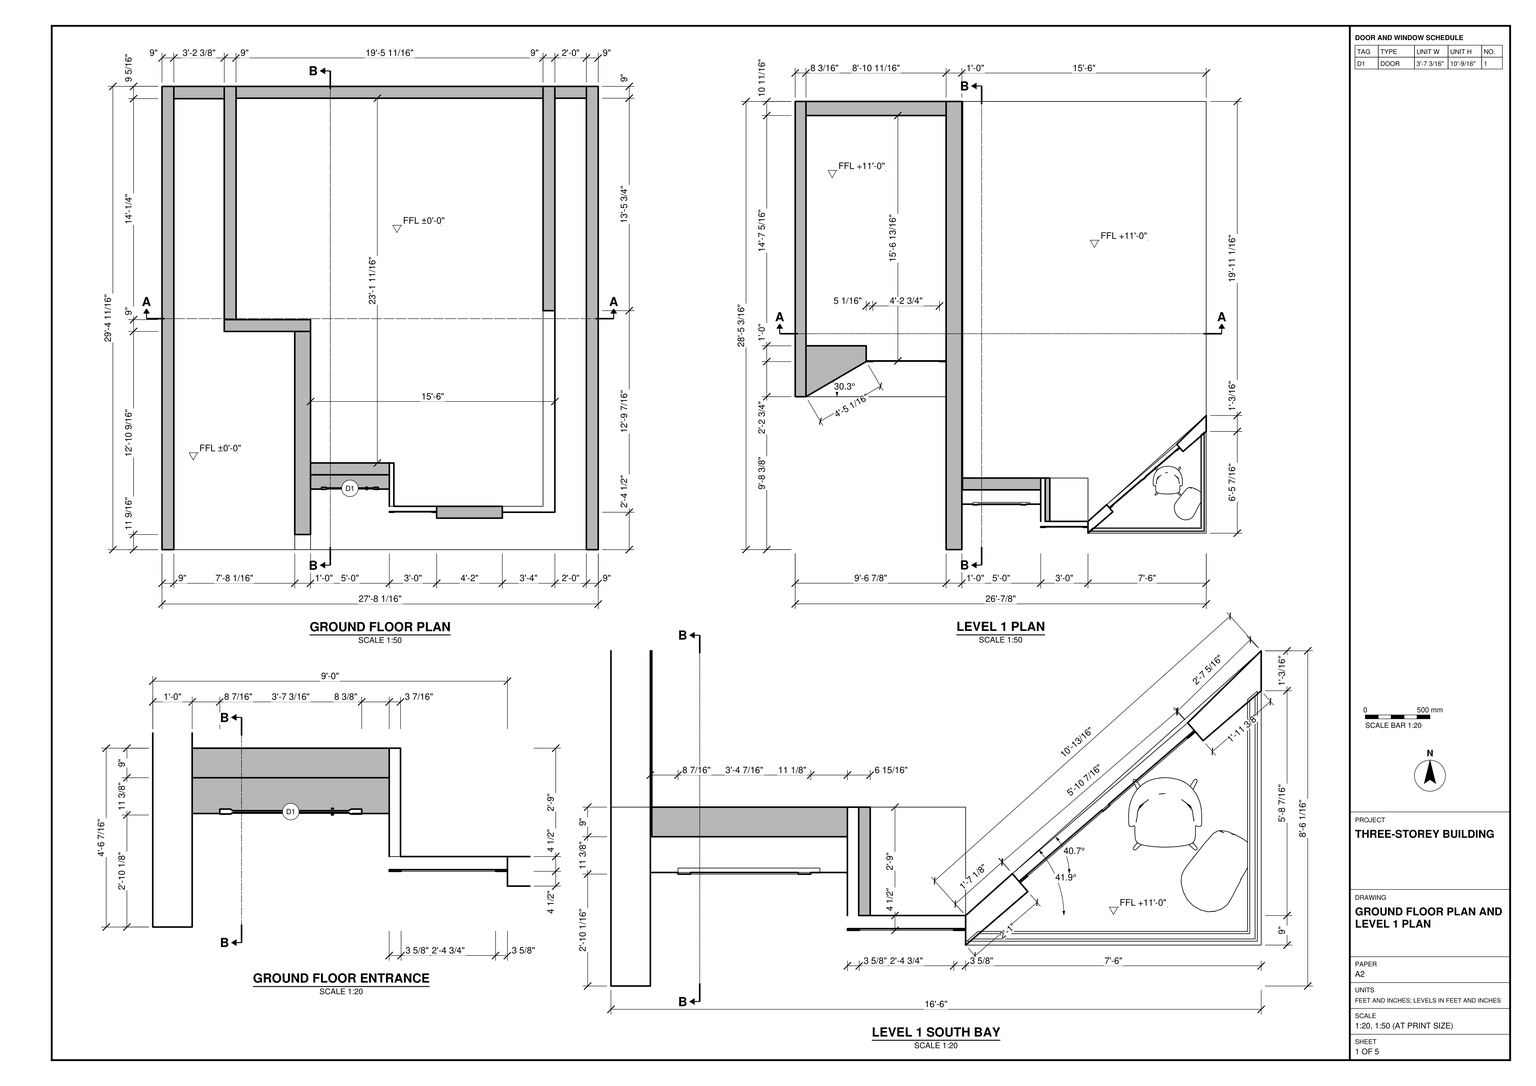
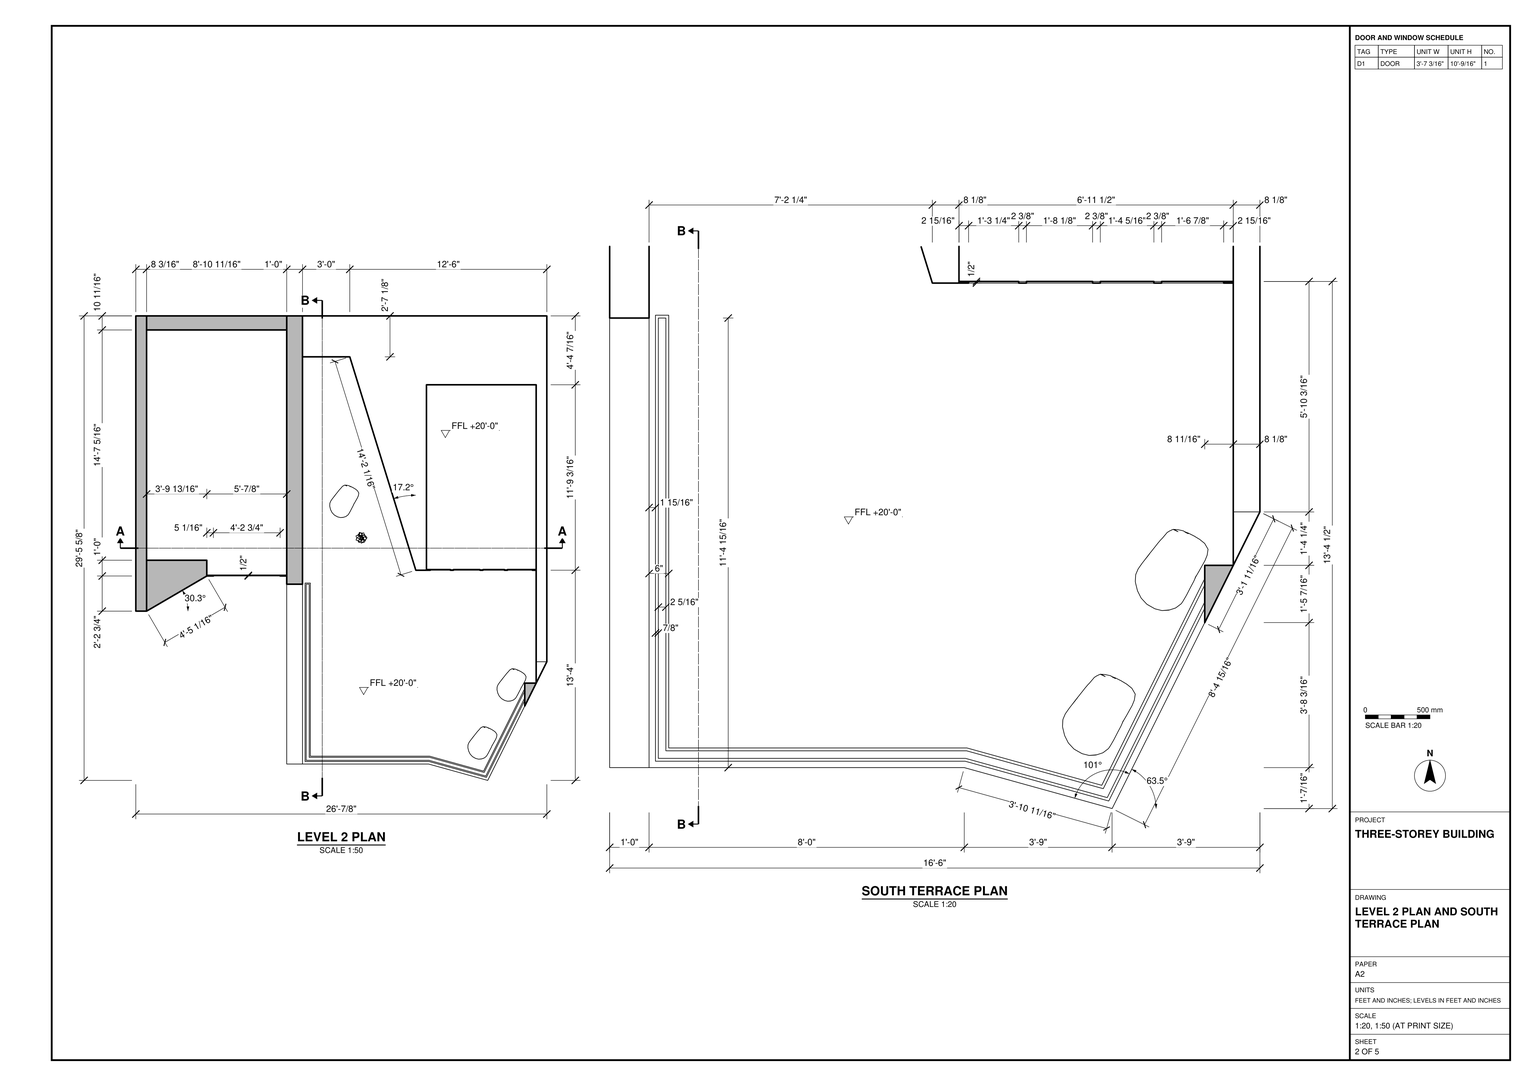
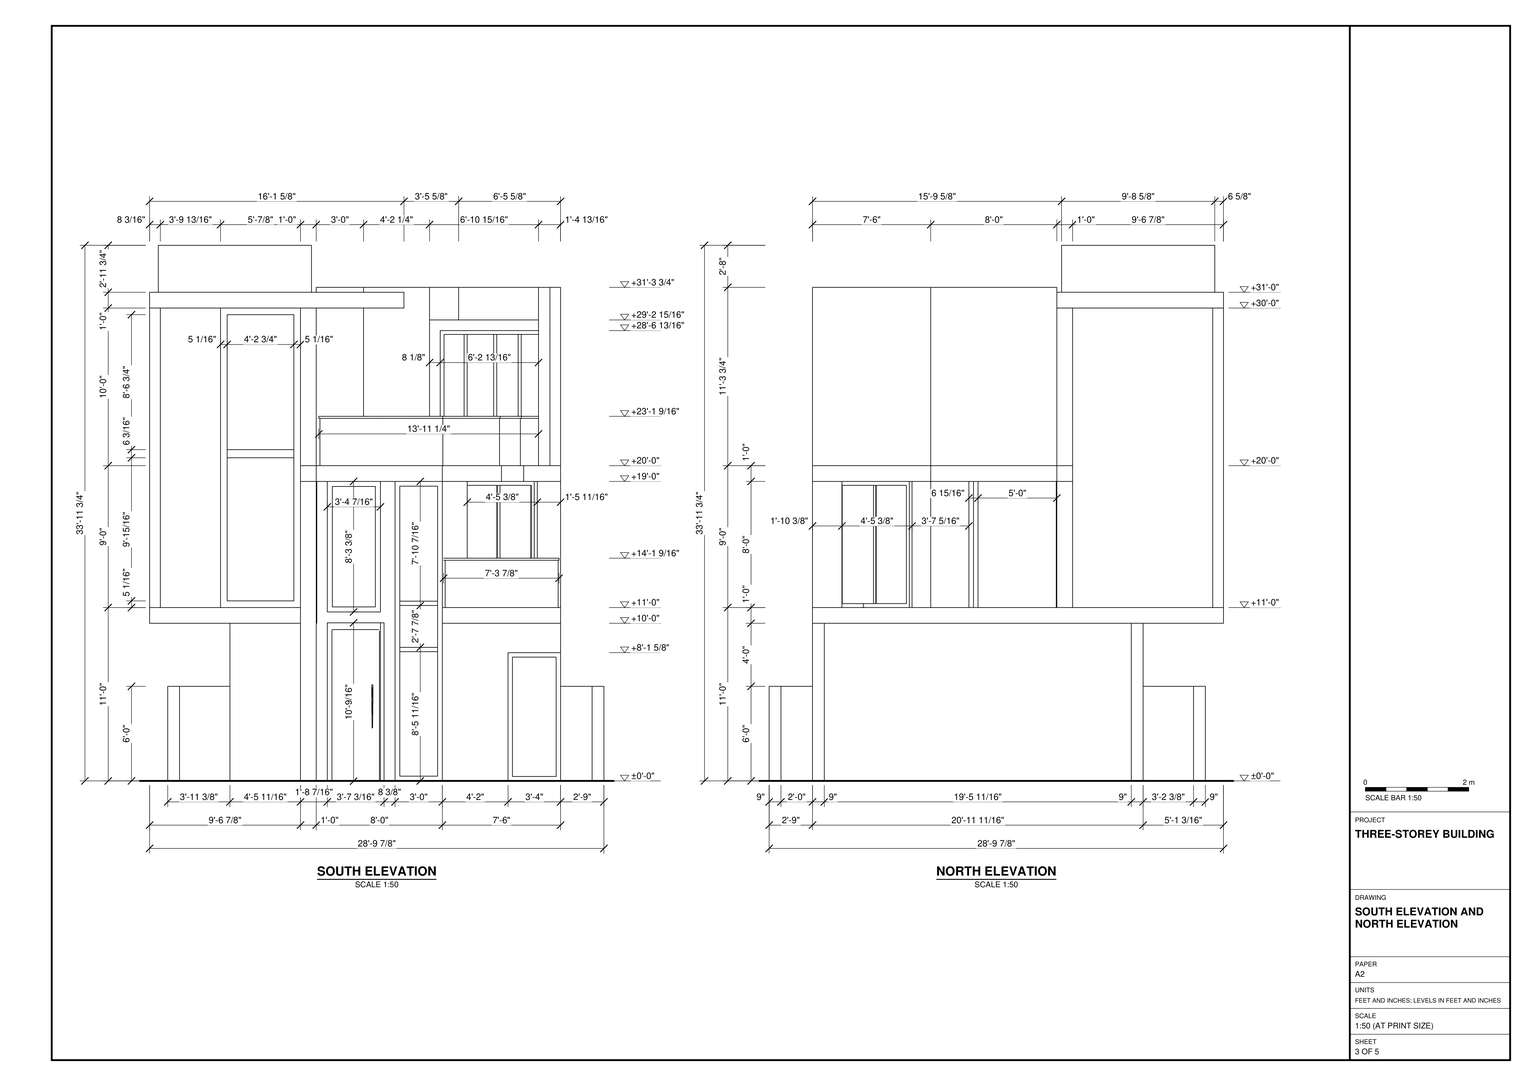
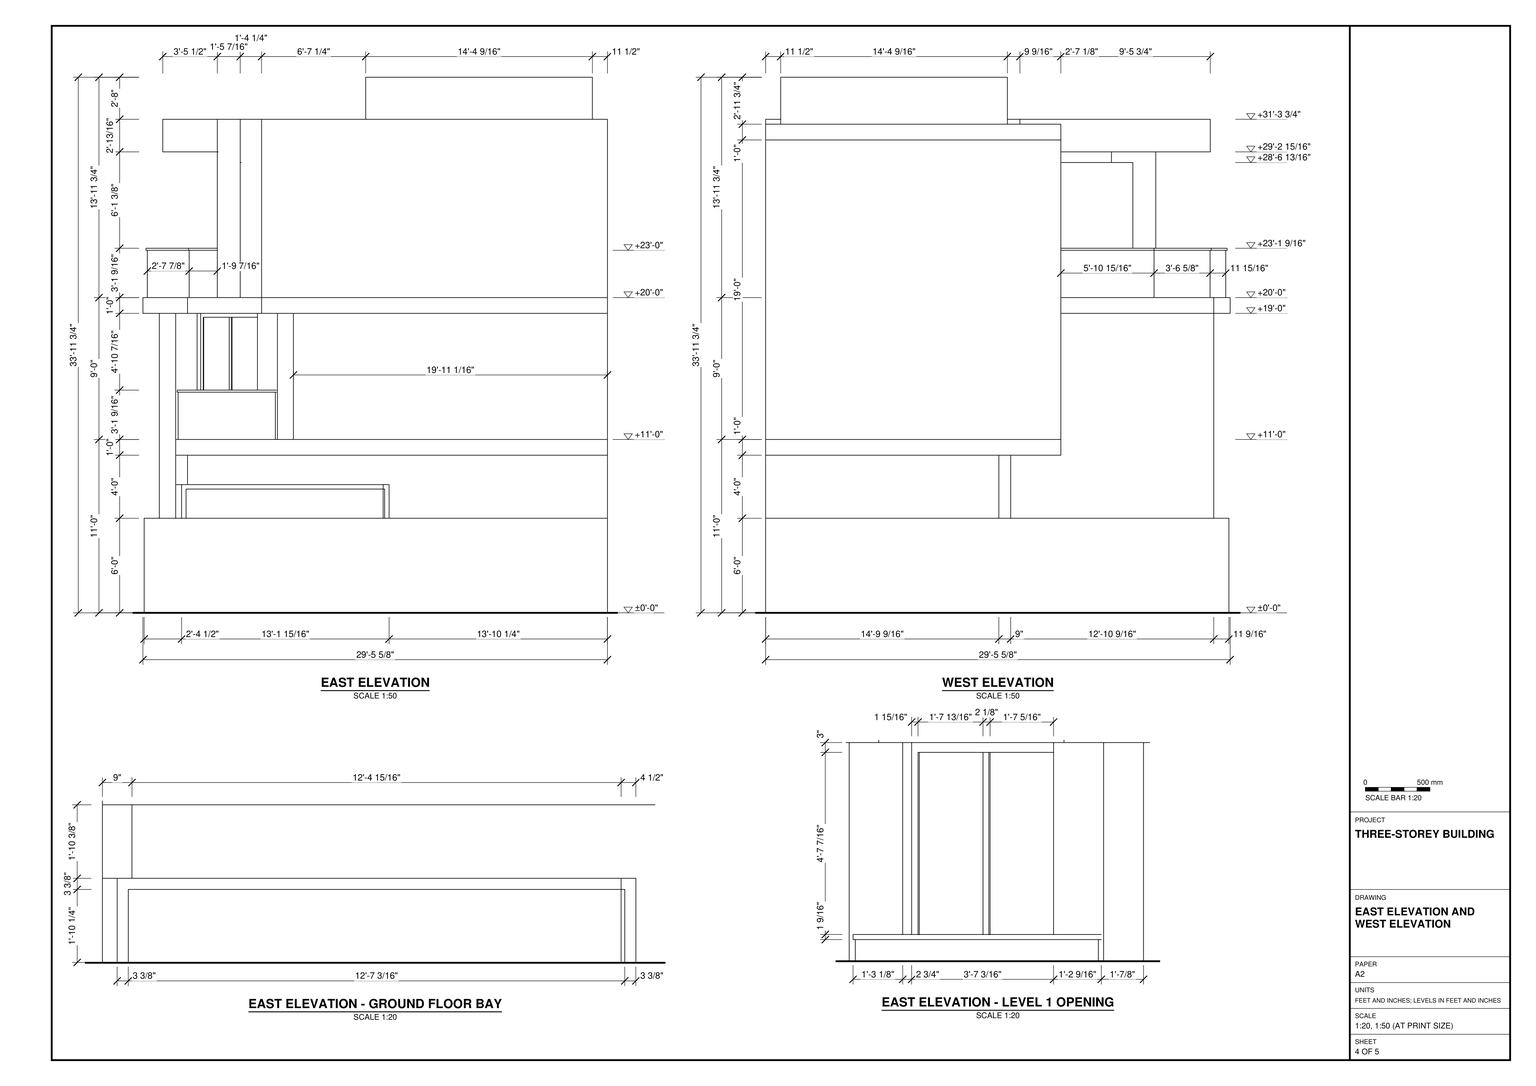
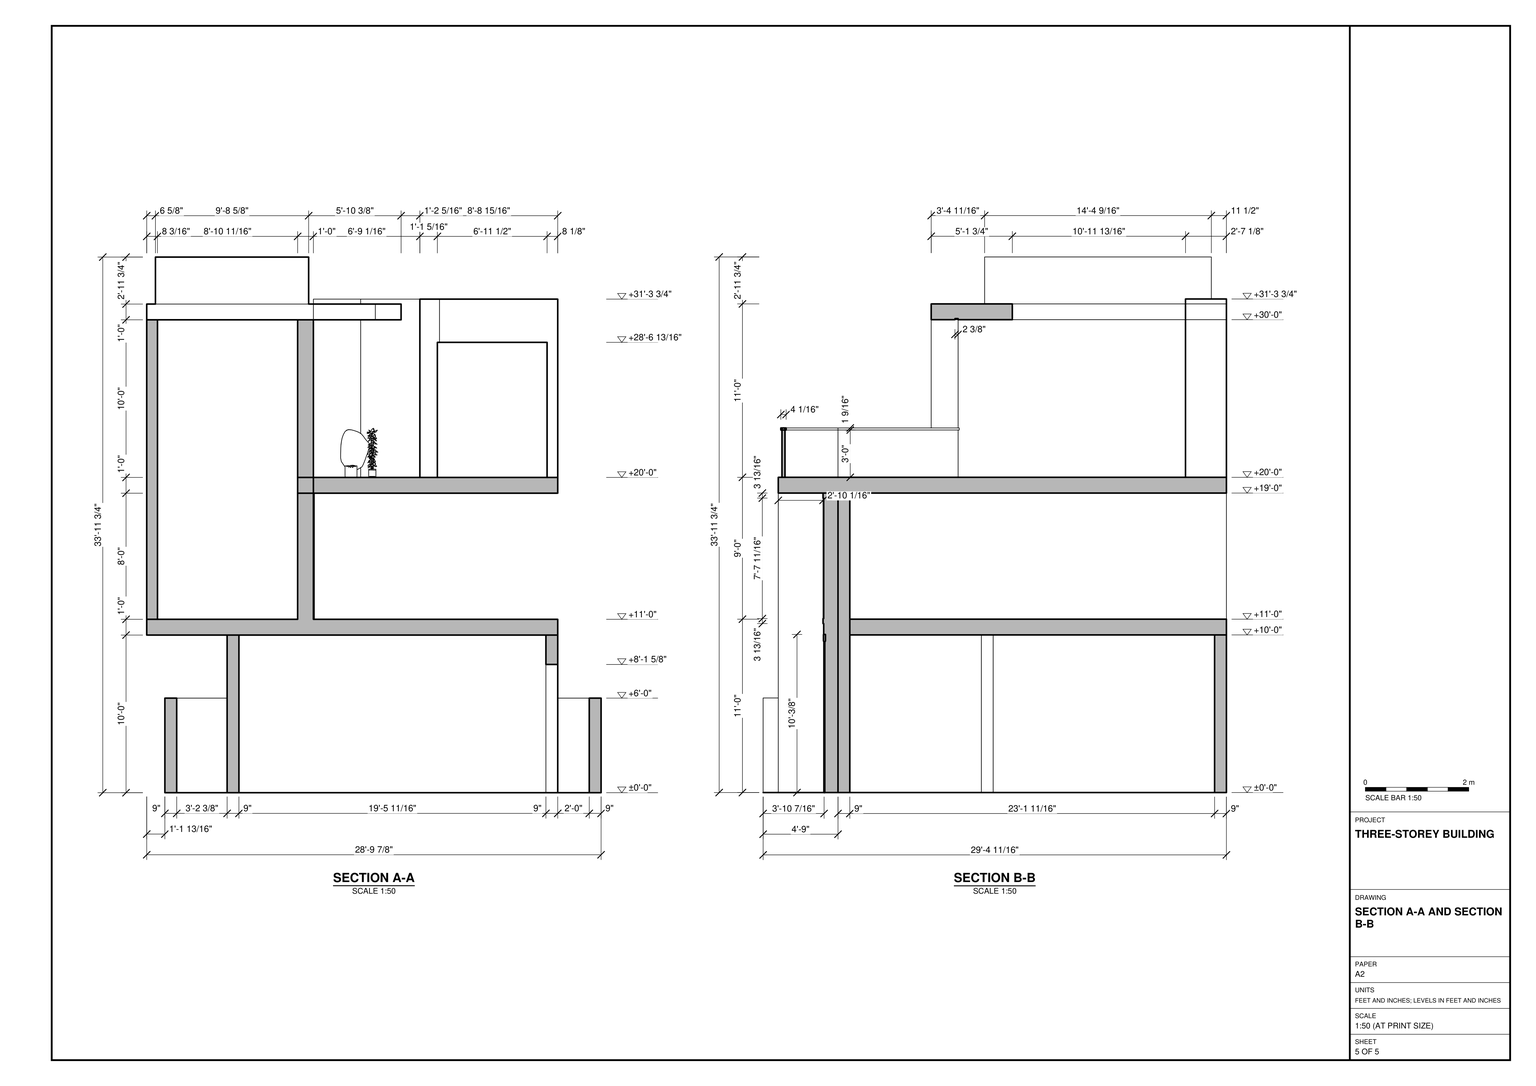
Build the three-storey building in SketchUp using task_files/diagram_01.pdf. Work in feet and inches. Set out the model with an overall width of 28'-9 7/8" along X, a depth of 29'-5 5/8" along Y and a height of 33'-11 15/16" along Z. Use finished floor levels of ±0'-0" for the ground floor, +11'-0" for Level 1 and +20'-0" for Level 2.

Follow the ground-floor plan for the long outer walls, the offset in the interior wall and the stepped south entrance. Use the wall thicknesses shown, including the 9" outer side walls at ground level. Fit the entrance door into its recess and use the elevations to align the framed openings with the slab edges. On Level 1, form the triangular south bay with its diagonal edge and seating. Above it, follow the Level 2 plan for the larger south terrace: its front edge changes direction before meeting the long angled side. Carry the terrace guard around those changes in direction. Model the flat roof sections at their different heights so the narrow western volume rises above the adjoining roof.

Keep walls, slabs, roof sections and each furniture or joinery piece in separate groups or components, and use components for repeated parts. Decor and loose items, including plants, may be any suitable library components. Save one SketchUp model as output_files/three_storey_building_with_a_faceted_south_terrace.skp.

# SketchUp Ruby script. Lengths in inches.
U = 1.inch
M = Sketchup.active_model
def pt(a) = Geom::Point3d.new(a.map { |v| v * U })
def face(e, loops, mat)
  f = e.add_face(loops[0].map { |a| pt(a) })
  loops[1..].each { |l| e.add_face(l.map { |a| pt(a) }).erase! }
  f.material = f.back_material = mat if mat
  f
end
# faces: each face lists its corners as indices into pts; further lists are holes
def faces(e, pts, list, mat = nil) = list.each { |f| face(e, (f[0].is_a?(Array) ? f : [f]).map { |l| l.map { |i| pts[i] } }, mat) }
# xy, xz, yz: faces in a plane at the given z, y or x. An outline is a flat list of corners, or four numbers for a rectangle; further outlines are holes
def ring(l) = l.size == 4 ? [[l[0], l[1]], [l[2], l[1]], [l[2], l[3]], [l[0], l[3]]] : l.each_slice(2).to_a
def flat(e, list, mat, &to3) = list.each { |f| face(e, (f[0].is_a?(Array) ? f : [f]).map { |l| ring(l).map { |u, v| to3.(u, v) } }, mat) }
def xy(e, z, list, mat = nil) = flat(e, list, mat) { |x, y| [x, y, z] }
def xz(e, y, list, mat = nil) = flat(e, list, mat) { |x, z| [x, y, z] }
def yz(e, x, list, mat = nil) = flat(e, list, mat) { |y, z| [x, y, z] }
def lines(e, pts, list) = list.each { |a, b| e.add_line(pt(pts[a]), pt(pts[b])) }
# prism: a flat outline (further loops are holes) pulled along v
def prism(e, loops, v, mat = nil)
  f = face(e, loops, mat); d = Geom::Vector3d.new(v.map { |x| x * U })
  f.pushpull(f.normal.samedirection?(d) ? d.length : -d.length)
end
def box(e, o, s, mat = nil) = prism(e, [[o, [o[0] + s[0], o[1], o[2]], [o[0] + s[0], o[1] + s[1], o[2]], [o[0], o[1] + s[1], o[2]]]], [0, 0, s[2]], mat)
def at(x, y, z, deg = 0) = Geom::Transformation.translation(pt([x, y, z])) * Geom::Transformation.rotation(ORIGIN, Z_AXIS, deg.degrees)
def axes(o, x, y, z) = Geom::Transformation.new([*x, 0, *y, 0, *z, 0, *pt(o).to_a, 1])
def part(name) = M.definitions.add(name)
# library, detail: a bought-in or finely detailed component or shape, given as its bounding box
def library(name, o, s) = part(name).tap { |d| box(d.entities, o, s) }
def detail(e, o, s) = box(e.add_group.entities, o, s)
def put(e, d, t, mat = nil) = e.add_instance(d, t).tap { |i| i.material = mat if mat }
def group(e, t, mat = nil) = e.add_group.tap { |g| g.transformation = t; g.material = mat if mat }.entities
root = M.entities
M.materials.add("[Color M06]").color = [86, 86, 86]
M.materials.add("[Color M07]").color = [58, 58, 58]
M.materials.add("[Mirror 02]").color = [229, 229, 229]
M.materials.add("[Wood Veneer 01]").color = [120, 70, 37]
c1 = library("Door 243 053",[-21.6,-2.79,-0.07],[43.2,5.58,82.64])
c2 = library("Chair 293 011 002",[-11.125,-11.03,-0.12],[22.25,22.06,31.4])
c3 = library("Ficus elastica Belize 002",[-7.92,-8.8125,0.01],[22.14,24.73,36.43])
c4 = library("Tall Climbing Plant 50-13",[-4.09,-3.9375,0],[8.41,8.24,37.49])
xy(root,0,[[13.8125,0.9375,22.8125,353.625],[22.8125,0.9375,114.875,0.9375,114.875,167.0625,61.1875,167.0625,61.1875,344.28,22.8125,344.28],[114.875,0.9375,126.875,12.47],[126.875,0.9375,336.875,0.9375,336.875,344.625,312.875,344.625,312.875,29.4375,272.88,29.4375,272.88,24.9375,222.875,24.9375,222.875,29.4375,186.875,29.4375,186.875,29.9375,222.875,29.9375,222.875,33.9375,186.875,33.9375,186.875,47.05,126.875,47.05],[336.875,0.9375,345.875,353.625],
  [114.875,12.47,126.875,167.0625],[222.875,24.9375,272.88,33.9375],[186.875,29.4375,190.32,29.9375],[190.32,29.4375,222.875,29.9375],[272.88,29.4375,312.875,29.4375,312.875,182.89,303.875,182.89,303.875,33.9375,272.88,33.9375],
  [190.32,33.9375,303.875,33.9375,303.875,344.625,70.1875,344.625,70.1875,176.0625,126.875,176.0625,126.875,66.9375,190.32,66.9375],[186.875,33.9375,190.32,66.9375],[126.875,47.05,186.875,57.9375],[126.875,57.9375,186.875,66.9375],[61.1875,167.0625,126.875,176.0625],
  [61.1875,176.0625,70.1875,353.625],[303.875,182.89,312.875,353.625],[22.8125,344.28,61.1875,353.625],[70.1875,344.625,303.875,353.625],[312.875,344.625,336.875,353.625]])
xy(root,3.61,[[190.49,29.4375,219.26,29.9375]])
xy(root,72,[[13.8125,0.9375,22.8125,353.625],[336.875,0.9375,345.875,353.625],[22.8125,344.28,61.1875,353.625],[312.875,344.625,336.875,353.625]])
xy(root,97.62,[[272.88,24.9375,312.875,29.4375],[272.88,29.4375,312.875,33.9375],[303.875,33.9375,312.875,182.89]])
xy(root,98.38,[[190.49,29.4375,219.26,29.9375]])
xy(root,101.67,[[190.49,29.4375,219.26,29.9375]],"[Color M06]")
xy(root,120,[[222.875,24.9375,303.875,33.9375],[303.875,24.9375,312.875,33.9375],[222.875,33.9375,222.875,66.9375,126.875,66.9375,126.875,176.0625,70.1875,176.0625,70.1875,344.625,303.875,344.625,303.875,33.9375],[190.32,33.9375,193.82,66.9375],[193.82,33.9375,222.875,66.9375],
  [303.875,33.9375,312.875,353.625],[126.875,57.9375,127.3125,66.9375],[0,128.875,70.1875,167.0625],[70.1875,128.875,114.875,167.0625],[0,167.0625,61.1875,176.0625],
  [61.1875,167.0625,70.1875,176.0625],[70.1875,167.0625,126.875,176.0625],[0,176.0625,61.1875,353.625],[61.1875,176.0625,70.1875,353.625],[70.1875,344.625,303.875,353.625]])
xy(root,128.625,[[135.29,46.55,175.73,47.05]])
xy(root,132,[[222.875,24.9375,222.875,33.9375,237.11,46.6875,312.875,114.56,290.48,92.63,237.11,46.6875,239.13,44.34,239.45,43.96,241.8,41.23,226.92,28.42,225.03,26.79],[222.875,24.9375,312.875,24.9375,312.875,102.4,311.02,100.8,311.02,26.79,225.03,26.79],[225.03,26.79,226.92,28.42,309.39,28.42,309.39,99.4,311.02,100.8,311.02,26.79],[226.92,28.42,309.39,28.42,309.39,99.4,295.18,87.17,292.83,89.9,239.45,43.96,241.8,41.23],[222.875,33.9375,237.11,46.6875,312.875,114.56,312.875,353.625,127.3125,353.625,127.3125,66.9375,222.875,66.9375],
  [239.45,43.96,239.13,44.34,292.51,90.28,292.83,89.9],[239.13,44.34,292.51,90.28,290.48,92.63,237.11,46.6875],[126.875,66.9375,127.3125,353.625],[295.18,87.17,292.83,89.9,292.51,90.28,290.48,92.63,312.875,114.56,312.875,102.4,311.02,100.8,309.39,99.4],[0,128.875,8.19,353.625],
  [8.19,128.875,114.875,128.875,114.875,155.62,54.02,155.62],[8.19,128.875,8.19,167.62,54.02,167.62,54.02,155.62],[54.02,156.12,114.875,156.12,114.875,342.92,8.19,342.92,8.19,167.62,54.02,167.62],[8.19,342.92,114.875,353.625]])
xy(root,132,[[54.02,155.62,114.875,156.12]],"[Color M06]")
xy(root,132.46,[[139.13,46.55,171.89,47.05]],"[Color M06]")
xy(root,133.57,[[190.49,29.4375,219.26,29.9375]])
xy(root,134.98,[[241.72,45.9,264.7,65.6875,264.375,66.07,241.39,46.28],[264.7,65.6875,266.76,67.46,266.4375,67.84,264.375,66.07],[266.76,67.46,290.57,87.95,290.25,88.33,266.4375,67.84]])
xy(root,136.86,[[190.49,29.4375,219.26,29.9375]],"[Color M06]")
xy(root,137.04,[[59.06,155.62,109.83,156.12]],"[Color M06]")
xy(root,168,[[225.03,26.79,226.92,28.42,309.39,28.42,309.39,99.4,311.02,100.8,311.02,26.79]])
xy(root,168,[[[223.21,26.12,226.67,29.09,308.72,29.09,308.72,99.71,311.69,102.27,311.69,26.12],[225.03,26.79,311.02,26.79,311.02,100.8,309.39,99.4,309.39,28.42,226.92,28.42]]],"[Color M07]")
xy(root,169.5625,[[[223.21,26.12,311.69,26.12,311.69,102.27,308.72,99.71,308.72,29.09,226.67,29.09],[225.03,26.79,226.92,28.42,309.39,28.42,309.39,99.4,311.02,100.8,311.02,26.79]],[225.03,26.79,311.02,26.79,311.02,100.8,309.39,99.4,309.39,28.42,226.92,28.42]],"[Color M07]")
xy(root,224.16,[[139.13,46.55,171.89,47.05]],"[Color M06]")
xy(root,224.39,[[190.49,29.4375,219.26,29.9375]],"[Color M06]")
xy(root,225.02,[[264.7,65.6875,264.375,66.07,266.4375,67.84,266.76,67.46]])
xy(root,225.02,[[241.72,45.9,241.39,46.28,264.375,66.07,264.7,65.6875],[266.76,67.46,266.4375,67.84,290.25,88.33,290.57,87.95]],"[Color M06]")
xy(root,228,[[[267.875,0,222.875,12.47,126.875,12.47,126.875,57.9375,186.875,57.9375,186.875,33.9375,222.875,33.9375,222.875,29.9375,186.875,29.9375,186.875,29.4375,222.875,29.4375,222.875,24.9375,233.33,33.9375,241.8,41.23,239.45,43.96,292.83,89.9,295.18,87.17,312.875,102.4,312.875,90.34,284.78,33.9375],[263.49,12.42,304.84,81.78,304.84,93.78,303.16,93.78,303.16,83.84,262.66,14.63,233.22,22.32,155.72,22.32,155.72,43.61,153.95,43.61,153.95,20.54,233.64,20.54],[135.29,46.55,175.73,47.05]],[114.875,12.47,126.875,353.625],[222.875,24.9375,233.33,33.9375,222.875,33.9375],[193.82,33.9375,193.82,66.9375,127.3125,66.9375,127.3125,353.625,312.875,353.625,312.875,114.56,237.11,46.6875,222.875,33.9375],[186.875,33.9375,190.32,57.9375],
  [190.32,33.9375,193.82,57.9375],[222.875,33.9375,233.33,33.9375,241.8,41.23,239.45,43.96,239.13,44.34,237.11,46.6875,290.48,92.63,312.875,114.56,237.11,46.6875],[239.13,44.34,237.11,46.6875,290.48,92.63,292.51,90.28],[126.875,57.9375,127.3125,353.625],[186.875,57.9375,190.32,66.9375],
  [190.32,57.9375,193.82,66.9375],[295.18,87.17,312.875,102.4,312.875,114.56,290.48,92.63,292.51,90.28,292.83,89.9]])
xy(root,228,[[186.875,29.4375,190.32,29.9375],[190.32,29.4375,222.875,29.9375],[239.45,43.96,292.83,89.9,292.51,90.28,239.13,44.34],[135.29,46.55,175.73,47.05]],"[Color M06]")
xy(root,229,[[263.49,12.42,233.64,20.54,153.95,20.54,153.95,43.61,155.72,43.61,155.72,22.32,233.22,22.32,262.66,14.63,303.16,83.84,303.16,93.78,304.84,93.78,304.84,81.78]])
xy(root,240,[[267.875,0,284.78,33.9375,296.08,56.625,296.08,62.9375,282.26,35.19,266.39,3.33,223.26,15.28,129.69,15.28,129.69,149.375,131.99,149.375,131.99,17.58,223.57,17.58,265.18,6.06,296.08,68.1,296.08,74.0625,304.77,74.0625,304.77,160.01,213.14,160.01,162.875,322.48,126.875,322.48,126.875,12.47,222.875,12.47],[266.39,3.33,223.26,15.28,129.69,15.28,129.69,149.375,131.99,149.375,131.99,17.58,223.57,17.58,265.18,6.06,296.08,68.1,296.08,62.9375,282.26,35.19],[114.875,12.47,126.875,149.375],[296.08,56.625,304.77,74.0625,296.08,74.0625],[304.77,74.0625,312.875,90.34,304.77,90.34],
  [304.77,90.34,304.77,301.2,221.24,301.2,221.24,160.01,213.14,160.01,162.875,322.48,126.875,322.48,126.875,353.625,312.875,353.625,312.875,90.34],[114.875,149.375,126.875,353.625],[221.24,160.01,304.77,160.51],[221.24,160.51,304.77,301.2]])
xy(root,242.92,[[224.17,160.01,239.44,160.51],[239.44,160.01,241.78,160.51],[241.78,160.01,261.94,160.51],[261.94,160.01,264.28,160.51],[264.28,160.01,280.59,160.51],
  [280.59,160.01,282.9375,160.51],[282.9375,160.01,301.84,160.51]])
xy(root,246,[[59.06,155.62,109.83,156.12]],"[Color M06]")
xy(root,252.1875,[[59.06,155.62,109.83,156.12]],"[Color M06]")
xy(root,276,[[266.39,3.33,223.26,15.28,129.69,15.28,129.69,149.375,131.99,149.375,131.99,17.58,223.57,17.58,265.18,6.06,296.08,68.1,296.08,62.9375,282.26,35.19]])
xy(root,276,[[[266.85,2.31,223.14,14.42,128.82,14.42,128.82,150.24,132.86,150.24,132.86,18.45,223.6875,18.45,264.72,7.08,296.95,71.79,296.95,62.73,283.04,34.81],[266.39,3.33,282.26,35.19,296.08,62.9375,296.08,68.1,265.18,6.06,223.57,17.58,131.99,17.58,131.99,149.375,129.69,149.375,129.69,15.28,223.26,15.28]]],"[Color M07]")
xy(root,277.5625,[[[266.85,2.31,283.04,34.81,296.95,62.73,296.95,71.79,264.72,7.08,223.6875,18.45,132.86,18.45,132.86,150.24,128.82,150.24,128.82,14.42,223.14,14.42],[266.39,3.33,223.26,15.28,129.69,15.28,129.69,149.375,131.99,149.375,131.99,17.58,223.57,17.58,265.18,6.06,296.08,68.1,296.08,62.9375,282.26,35.19]],[266.39,3.33,282.26,35.19,296.08,62.9375,296.08,68.1,265.18,6.06,223.57,17.58,131.99,17.58,131.99,149.375,129.69,149.375,129.69,15.28,223.26,15.28]],"[Color M07]")
xy(root,339.91,[[224.17,160.01,239.44,160.51],[239.44,160.01,241.78,160.51],[241.78,160.01,261.94,160.51],[261.94,160.01,264.28,160.51],[264.28,160.01,280.59,160.51],
  [280.59,160.01,282.9375,160.51],[282.9375,160.01,301.84,160.51]])
xy(root,342.84,[[296.08,74.0625,304.77,90.34],[221.24,160.51,304.77,301.2]])
xy(root,342.84,[[221.24,160.01,304.77,160.51]],"[Color M07]")
xy(root,350.94,[[[235.26,15.1,233.42,27.125,243.12,33.61,251.78,39.4,259.68,44.68,266.32,49.125,272.87,53.51,277.23,56.42,281.76,59.45,286.07,62.33,289.55,64.66,296.08,69.02,296.08,56.625],[238.58,23.8,277.55,50.41,276.88,51.39,237.91,24.79]],[233.42,27.125,213.14,160.01,225.23,160.01,243.12,33.61],[251.78,39.4,235.38,160.01,244.8125,160.01,259.68,44.68],[266.32,49.125,253.4,160.01,261.21,160.01,272.87,53.51],[277.23,56.42,267.7,160.01,274.17,160.01,281.76,59.45],
  [286.07,62.33,280.96,160.01,289.55,160.01,289.55,64.66],[296.08,90.34,297.16,160.01,304.77,160.01,304.77,90.34]])
xy(root,351.57,[[238.58,23.8,237.91,24.79,276.88,51.39,277.55,50.41]])
xy(root,354.96,[[59.06,155.62,109.83,156.12]],"[Color M06]")
xy(root,360,[[0,128.875,8.19,353.625],[8.19,128.875,54.02,155.62,114.875,155.62,114.875,128.875],[8.19,128.875,8.19,167.62,54.02,167.62,54.02,155.62],[114.875,128.875,193.625,128.875,193.625,149.375,174.04,149.375,174.04,146.98,132.51,146.98,132.51,149.375,114.875,149.375],[114.875,149.375,126.875,353.625],
  [126.875,149.375,126.875,190.64,174.02,190.64,174.02,286.14,193.625,286.14,193.625,149.375],[54.02,156.12,54.02,167.62,8.19,167.62,8.19,342.92,114.875,342.92,114.875,156.12],[8.19,342.92,114.875,353.625]])
xy(root,360,[[54.02,155.62,114.875,156.12]],"[Color M06]")
xy(root,360.8125,[[132.51,146.98,174.04,149.375]])
xy(root,372,[[[0,128.875,193.625,128.875,193.625,286.14,174.02,286.14,174.02,190.64,126.875,190.64,126.875,353.625,0,353.625],[6.63,169.58,123.26,342.14]]])
xy(root,375.75,[[[235.26,15.1,296.08,56.625,304.77,74.0625,312.875,90.34,312.875,353.625,126.875,353.625,126.875,322.48,162.875,322.48,213.14,160.01],[243.12,33.61,225.23,160.01,235.38,160.01,251.78,39.4],[259.68,44.68,244.8125,160.01,253.4,160.01,266.32,49.125],[289.55,64.66,289.55,160.01,297.16,160.01,296.08,90.34,296.08,69.02],[272.87,53.51,261.21,160.01,267.7,160.01,277.23,56.42],[281.76,59.45,274.17,160.01,280.96,160.01,286.07,62.33]]])
xy(root,407.75,[[6.63,169.58,123.26,342.14]])
xz(root,0.9375,[[13.8125,0,22.8125,72],[336.875,0,345.875,72]])
xz(root,12.47,[[114.875,0,126.875,228],[114.875,228,126.875,240],[126.875,228,222.875,240]])
xz(root,14.42,[[128.82,276,223.14,277.5625]],"[Color M07]")
xz(root,15.28,[[129.69,276,223.26,277.5625]])
xz(root,15.28,[[129.69,240,223.26,276]],"[Mirror 02]")
xz(root,17.58,[[131.99,276,223.57,277.5625]])
xz(root,17.58,[[131.99,240,223.57,276]],"[Mirror 02]")
xz(root,18.45,[[132.86,276,223.6875,277.5625]],"[Color M07]")
xz(root,20.54,[[153.95,228,233.64,229]])
xz(root,22.32,[[155.72,228,233.22,229]])
xz(root,24.9375,[[222.875,0,272.88,0,272.88,97.62,312.875,97.62,312.875,120,222.875,120],[222.875,120,312.875,132]])
xz(root,26.12,[[223.21,168,311.69,169.5625]],"[Color M07]")
xz(root,26.79,[[225.03,168,311.02,169.5625]])
xz(root,26.79,[[225.03,132,311.02,168]],"[Mirror 02]")
xz(root,28.42,[[226.92,168,309.39,169.5625]])
xz(root,28.42,[[226.92,132,309.39,168]],"[Mirror 02]")
xz(root,29.09,[[226.67,168,308.72,169.5625]],"[Color M07]")
xz(root,29.4375,[[[186.875,0,222.875,228],[190.49,3.61,219.26,224.39]],[[272.88,0,312.875,97.62],[276.24,3.37,309.51,94.25]],[190.49,98.38,219.26,101.67],[190.49,133.57,219.26,136.86]],"[Color M06]")
xz(root,29.4375,[[276.24,3.37,309.51,94.25]],"[Mirror 02]")
xz(root,29.9375,[[[186.875,0,222.875,228],[190.49,3.61,219.26,224.39]]])
xz(root,29.9375,[[190.49,3.61,219.26,98.38],[190.49,101.67,219.26,133.57],[190.49,136.86,219.26,224.39]],"[Mirror 02]")
xz(root,33.9375,[[190.32,0,222.875,120],[222.875,0,222.875,120,303.875,120,303.875,97.62,272.88,97.62,272.88,0],[190.32,120,193.82,228],[193.82,120,222.875,228]])
xz(root,43.61,[[153.95,228,155.72,229]])
xz(root,46.55,[[[135.29,128.625,175.73,228],[139.13,132.46,171.89,224.16]]],"[Color M06]")
xz(root,47.05,[[139.13,132.46,171.89,224.16]],"[Mirror 02]")
xz(root,47.05,[[126.875,0,135.29,0,135.29,120.36,175.73,120.36,175.73,0,186.875,0,186.875,228,175.73,228,175.73,128.625,135.29,128.625,135.29,228,127.3125,228,127.3125,120,126.875,120]],"[Wood Veneer 01]")
xz(root,57.9375,[[126.875,0,186.875,0,186.875,228,127.3125,228,127.3125,120,126.875,120],[126.875,120,127.3125,228]])
xz(root,66.9375,[[126.875,0,186.875,120],[186.875,0,190.32,120],[126.875,120,127.3125,132],[127.3125,120,186.875,132],[186.875,120,190.32,132],
  [190.32,120,193.82,132],[193.82,120,222.875,132],[127.3125,132,186.875,228],[186.875,132,190.32,228],[190.32,132,193.82,228]])
xz(root,74.0625,[[296.08,240,304.77,342.84]])
xz(root,90.34,[[296.08,342.84,304.77,350.94]])
xz(root,93.78,[[303.16,228,304.84,229]])
xz(root,128.875,[[0,120,114.875,132],[0,132,8.19,360],[0,360,193.625,372]])
xz(root,146.98,[[132.51,360,174.04,360.8125]])
xz(root,149.375,[[114.875,240,126.875,360],[129.69,240,131.99,276],[129.69,276,131.99,277.5625],[132.51,360,174.04,360.8125]])
xz(root,150.24,[[128.82,276,132.86,277.5625]])
xz(root,155.62,[[[54.02,132,114.875,360],[59.06,137.04,109.83,354.96]],[59.06,246,109.83,252.1875]],"[Color M06]")
xz(root,156.12,[[[54.02,132,114.875,360],[59.06,137.04,109.83,354.96]]])
xz(root,156.12,[[59.06,137.04,109.83,246],[59.06,252.1875,109.83,354.96]],"[Mirror 02]")
xz(root,160.01,[[213.14,240,221.24,240,221.24,342.84,304.77,342.84,304.77,350.94,297.16,350.94,297.16,375.75,289.55,375.75,289.55,350.94,280.96,350.94,280.96,375.75,274.17,375.75,274.17,350.94,267.7,350.94,267.7,375.75,261.21,375.75,261.21,350.94,253.4,350.94,253.4,375.75,244.8125,375.75,244.8125,350.94,235.38,350.94,235.38,375.75,225.23,375.75,225.23,350.94,213.14,350.94]])
xz(root,160.01,[[[221.24,240,304.77,342.84],[224.17,242.92,301.84,339.91]],[239.44,242.92,241.78,339.91],[261.94,242.92,264.28,339.91],[280.59,242.92,282.9375,339.91]],"[Color M07]")
xz(root,160.51,[[[221.24,240,304.77,342.84],[224.17,242.92,301.84,339.91]]])
xz(root,160.51,[[224.17,242.92,239.44,339.91],[241.78,242.92,261.94,339.91],[264.28,242.92,280.59,339.91],[282.9375,242.92,301.84,339.91]],"[Mirror 02]")
xz(root,167.0625,[[61.1875,0,114.875,120],[114.875,0,126.875,120]])
xz(root,167.62,[[8.19,132,54.02,360]])
xz(root,169.58,[[6.63,372,123.26,407.75]])
xz(root,176.0625,[[61.1875,0,70.1875,120],[70.1875,0,126.875,120]])
xz(root,182.89,[[303.875,0,312.875,97.62]])
xz(root,190.64,[[126.875,360,174.02,372]])
xz(root,286.14,[[174.02,360,193.625,372]])
xz(root,301.2,[[221.24,240,304.77,342.84]])
xz(root,322.48,[[126.875,240,162.875,375.75]])
xz(root,342.14,[[6.63,372,123.26,407.75]])
xz(root,342.92,[[8.19,132,114.875,360]])
xz(root,344.28,[[22.8125,0,61.1875,72]])
xz(root,344.625,[[70.1875,0,303.875,120],[312.875,0,336.875,72]])
xz(root,353.625,[[13.8125,0,22.8125,72],[22.8125,0,61.1875,72],[61.1875,0,70.1875,120],[70.1875,0,303.875,120],[303.875,0,312.875,120],
  [312.875,0,336.875,72],[336.875,0,345.875,72],[0,120,312.875,132],[0,132,8.19,360],[8.19,132,114.875,360],
  [114.875,132,126.875,228],[126.875,132,127.3125,228],[114.875,228,126.875,240],[126.875,228,222.875,240],[222.875,228,312.875,240],
  [114.875,240,126.875,360],[126.875,240,222.875,375.75],[222.875,240,312.875,375.75],[0,360,126.875,372]])
yz(root,0,[[128.875,120,353.625,132],[128.875,132,353.625,360],[128.875,360,353.625,372]])
yz(root,6.63,[[169.58,372,342.14,407.75]])
yz(root,8.19,[[128.875,132,167.62,360],[167.62,132,342.92,360],[342.92,132,353.625,360]])
yz(root,13.8125,[[0.9375,0,353.625,72]])
yz(root,22.8125,[[0.9375,0,344.28,72],[344.28,0,353.625,72]])
yz(root,54.02,[[156.12,132,167.62,360]])
yz(root,54.02,[[155.62,132,156.12,360]],"[Color M06]")
yz(root,59.06,[[155.62,246,156.12,252.1875]])
yz(root,59.06,[[155.62,137.04,156.12,246],[155.62,252.1875,156.12,354.96]],"[Color M06]")
yz(root,61.1875,[[167.0625,0,176.0625,120],[176.0625,0,176.0625,120,353.625,120,353.625,72,344.28,72,344.28,0],[344.28,0,353.625,72]])
yz(root,70.1875,[[176.0625,0,344.625,120],[344.625,0,353.625,120]])
yz(root,109.83,[[155.62,246,156.12,252.1875]])
yz(root,109.83,[[155.62,137.04,156.12,228],[155.62,228,156.12,240],[155.62,240,156.12,246],[155.62,252.1875,156.12,354.96]],"[Color M06]")
yz(root,114.875,[[12.47,0,12.47,228,155.62,228,155.62,132,128.875,132,128.875,120,167.0625,120,167.0625,0],[156.12,132,342.92,228],[342.92,132,353.625,228],[12.47,228,155.62,240],[155.62,228,156.12,240],
  [156.12,228,342.92,240],[342.92,228,353.625,240],[149.375,240,155.62,360],[155.62,240,156.12,360],[156.12,240,342.92,360],
  [342.92,240,353.625,360]])
yz(root,114.875,[[155.62,132,156.12,228]],"[Color M06]")
yz(root,123.26,[[169.58,372,342.14,407.75]])
yz(root,126.875,[[12.47,0,57.9375,228],[57.9375,0,66.9375,120],[66.9375,0,167.0625,120],[167.0625,0,176.0625,120],[57.9375,120,57.9375,228,353.625,228,353.625,132,66.9375,132,66.9375,120],
  [12.47,228,57.9375,240],[57.9375,228,353.625,240],[149.375,240,322.48,360],[322.48,240,353.625,360],[190.64,360,322.48,372],
  [322.48,360,353.625,372],[322.48,372,353.625,375.75]])
yz(root,127.3125,[[57.9375,120,66.9375,228],[66.9375,132,353.625,228]])
yz(root,128.82,[[14.42,276,57.9375,277.5625],[57.9375,276,150.24,277.5625]],"[Color M07]")
yz(root,129.69,[[15.28,276,57.9375,277.5625],[57.9375,276,149.375,277.5625]])
yz(root,129.69,[[15.28,240,57.9375,276],[57.9375,240,149.375,276]],"[Mirror 02]")
yz(root,131.99,[[17.58,276,57.9375,277.5625],[57.9375,276,149.375,277.5625]])
yz(root,131.99,[[17.58,240,57.9375,276],[57.9375,240,149.375,276]],"[Mirror 02]")
yz(root,132.51,[[146.98,360,149.375,360.8125]])
yz(root,132.86,[[18.45,276,57.9375,277.5625],[57.9375,276,150.24,277.5625]],"[Color M07]")
yz(root,135.29,[[46.55,128.625,47.05,228]],"[Color M06]")
yz(root,139.13,[[46.55,132.46,47.05,224.16]],"[Color M06]")
yz(root,153.95,[[20.54,228,43.61,229]])
yz(root,155.72,[[22.32,228,43.61,229]])
yz(root,171.89,[[46.55,132.46,47.05,224.16]],"[Color M06]")
yz(root,174.02,[[190.64,360,286.14,372]])
yz(root,174.04,[[146.98,360,149.375,360.8125]])
yz(root,175.73,[[46.55,128.625,47.05,228]])
yz(root,186.875,[[33.9375,0,47.05,228],[47.05,0,57.9375,228],[57.9375,0,66.9375,120],[57.9375,120,66.9375,228]])
yz(root,186.875,[[29.4375,0,29.9375,228]],"[Color M06]")
yz(root,190.32,[[33.9375,0,66.9375,120],[33.9375,120,66.9375,228]])
yz(root,190.49,[[29.4375,98.38,29.9375,101.67],[29.4375,133.57,29.9375,136.86]])
yz(root,190.49,[[29.4375,3.61,29.9375,98.38],[29.4375,101.67,29.9375,133.57],[29.4375,136.86,29.9375,224.39]],"[Color M06]")
yz(root,193.625,[[128.875,360,286.14,372]])
yz(root,193.82,[[33.9375,120,66.9375,228]])
yz(root,219.26,[[29.4375,3.61,29.9375,98.38],[29.4375,98.38,29.9375,101.67],[29.4375,133.57,29.9375,136.86]])
yz(root,219.26,[[29.4375,101.67,29.9375,120],[29.4375,120,29.9375,132],[29.4375,132,29.9375,133.57],[29.4375,136.86,29.9375,224.39]],"[Color M06]")
yz(root,221.24,[[160.01,240,160.51,342.84],[160.51,240,301.2,342.84]])
yz(root,222.875,[[24.9375,0,29.4375,120],[29.9375,0,33.9375,120],[24.9375,120,29.4375,132],[29.9375,120,33.9375,132],[33.9375,120,66.9375,132],
  [24.9375,132,29.4375,228],[29.9375,132,33.9375,228]])
yz(root,222.875,[[29.4375,0,29.9375,120],[29.4375,120,29.9375,132],[29.4375,132,29.9375,228]],"[Color M06]")
yz(root,224.17,[[160.01,242.92,160.51,339.91]],"[Color M07]")
yz(root,239.44,[[160.01,242.92,160.51,339.91]],"[Color M07]")
yz(root,241.78,[[160.01,242.92,160.51,339.91]],"[Color M07]")
yz(root,261.94,[[160.01,242.92,160.51,339.91]],"[Color M07]")
yz(root,264.28,[[160.01,242.92,160.51,339.91]],"[Color M07]")
yz(root,272.88,[[24.9375,0,29.4375,97.62],[29.4375,0,33.9375,97.62]])
yz(root,280.59,[[160.01,242.92,160.51,339.91]],"[Color M07]")
yz(root,282.9375,[[160.01,242.92,160.51,339.91]],"[Color M07]")
yz(root,289.55,[[64.66,350.94,160.01,375.75]])
yz(root,296.08,[[56.625,240,56.625,350.94,69.02,350.94,69.02,375.75,90.34,375.75,90.34,342.84,74.0625,342.84,74.0625,240,68.1,240,68.1,277.5625,62.9375,277.5625,62.9375,240],[62.9375,240,68.1,276],[62.9375,276,68.1,277.5625]])
yz(root,296.95,[[62.73,276,71.79,277.5625]])
yz(root,301.84,[[160.01,242.92,160.51,339.91]],"[Color M07]")
yz(root,303.16,[[83.84,228,93.78,229]])
yz(root,303.875,[[182.89,0,182.89,97.62,33.9375,97.62,33.9375,120,344.625,120,344.625,0],[344.625,0,353.625,120]])
yz(root,304.77,[[74.0625,240,160.01,342.84],[160.51,240,301.2,342.84],[90.34,342.84,160.01,350.94]])
yz(root,304.77,[[160.01,240,160.51,342.84]],"[Color M07]")
yz(root,304.84,[[81.78,228,93.78,229]])
yz(root,308.72,[[29.09,168,99.71,169.5625]],"[Color M07]")
yz(root,309.39,[[28.42,168,99.4,169.5625]])
yz(root,309.39,[[28.42,132,99.4,168]],"[Mirror 02]")
yz(root,311.02,[[26.79,168,100.8,169.5625]])
yz(root,311.02,[[26.79,132,100.8,168]],"[Mirror 02]")
yz(root,311.69,[[26.12,168,102.27,169.5625]],"[Color M07]")
yz(root,312.875,[[187.39,0,344.625,0,344.625,72,353.625,72,353.625,120,33.9375,120,33.9375,97.62,187.39,97.62],[182.89,0,187.39,0,187.39,97.62,182.89,97.62,182.89,94.24,184,94.24,184,3.38,182.89,3.38],[344.625,0,353.625,72],[24.9375,97.62,33.9375,120],[24.9375,120,353.625,132],
  [102.4,132,114.56,228],[90.34,228,353.625,240],[90.34,240,353.625,375.75]])
yz(root,312.875,[[[29.4375,0,187.39,97.62],[32.82,3.38,184,94.24]]],"[Color M06]")
yz(root,312.875,[[32.82,3.38,182.89,94.24],[182.89,3.38,184,94.24]],"[Mirror 02]")
yz(root,336.875,[[0.9375,0,344.625,72],[344.625,0,353.625,72]])
yz(root,345.875,[[0.9375,0,353.625,72]])
p = [[222.875,24.9375,132],[225.03,26.79,132],[225.03,26.79,168],[225.03,26.79,169.5625],[226.92,28.42,169.5625],[226.92,28.42,168],
  [226.92,28.42,132],[241.8,41.23,132],[241.8,41.23,228],[233.33,33.9375,228],[222.875,24.9375,228],[222.875,33.9375,228],
  [237.11,46.6875,228],[237.11,46.6875,132],[222.875,33.9375,132],[239.45,43.96,132],[239.45,43.96,228],[239.13,44.34,228],
  [239.13,44.34,132],[292.83,89.9,132],[292.83,89.9,228],[266.76,67.46,225.02],[290.57,87.95,225.02],[290.57,87.95,134.98],
  [266.76,67.46,134.98],[264.7,65.6875,134.98],[241.72,45.9,134.98],[241.72,45.9,225.02],[264.7,65.6875,225.02],[292.51,90.28,132],
  [292.51,90.28,228],[290.25,88.33,225.02],[266.4375,67.84,225.02],[264.375,66.07,225.02],[241.39,46.28,225.02],[241.39,46.28,134.98],
  [264.375,66.07,134.98],[266.4375,67.84,134.98],[290.25,88.33,134.98],[295.18,87.17,228],[295.18,87.17,132],[312.875,102.4,228],
  [309.39,99.4,132],[309.39,99.4,168],[309.39,99.4,169.5625],[311.02,100.8,169.5625],[311.02,100.8,168],[311.02,100.8,132],
  [312.875,102.4,132],[290.48,92.63,132],[290.48,92.63,228],[312.875,114.56,132],[312.875,114.56,228],[8.19,128.875,132],
  [54.02,155.62,132],[54.02,155.62,360],[8.19,128.875,360],[226.67,29.09,168],[223.21,26.12,168],[223.21,26.12,169.5625],
  [226.67,29.09,169.5625],[311.69,102.27,168],[308.72,99.71,168],[308.72,99.71,169.5625],[311.69,102.27,169.5625],[222.875,12.47,228],
  [267.875,0,228],[267.875,0,240],[222.875,12.47,240],[284.78,33.9375,228],[284.78,33.9375,240],[263.49,12.42,228],
  [233.64,20.54,228],[233.64,20.54,229],[263.49,12.42,229],[304.84,81.78,228],[304.84,81.78,229],[233.22,22.32,228],
  [262.66,14.63,228],[262.66,14.63,229],[233.22,22.32,229],[303.16,83.84,228],[303.16,83.84,229],[312.875,90.34,228],
  [312.875,90.34,240],[304.77,74.0625,240],[296.08,56.625,240],[223.26,15.28,240],[266.39,3.33,240],[266.39,3.33,276],
  [223.26,15.28,276],[282.26,35.19,240],[282.26,35.19,276],[265.18,6.06,240],[223.57,17.58,240],[223.57,17.58,276],
  [265.18,6.06,276],[296.08,68.1,240],[296.08,68.1,276],[296.08,62.9375,240],[296.08,62.9375,276],[304.77,74.0625,342.84],
  [304.77,74.0625,375.75],[296.08,56.625,375.75],[296.08,56.625,350.94],[312.875,90.34,375.75],[162.875,322.48,240],[213.14,160.01,240],
  [213.14,160.01,350.94],[213.14,160.01,375.75],[162.875,322.48,375.75],[223.14,14.42,276],[266.85,2.31,276],[266.85,2.31,277.5625],
  [223.14,14.42,277.5625],[283.04,34.81,276],[283.04,34.81,277.5625],[266.39,3.33,277.5625],[223.26,15.28,277.5625],[282.26,35.19,277.5625],
  [223.57,17.58,277.5625],[265.18,6.06,277.5625],[296.08,68.1,277.5625],[264.72,7.08,276],[223.6875,18.45,276],[223.6875,18.45,277.5625],
  [264.72,7.08,277.5625],[296.95,71.79,276],[296.95,71.79,277.5625],[296.95,62.73,276],[296.95,62.73,277.5625],[296.08,62.9375,277.5625],
  [235.26,15.1,375.75],[233.42,27.125,350.94],[235.26,15.1,350.94],[238.58,23.8,350.94],[237.91,24.79,350.94],[237.91,24.79,351.57],
  [238.58,23.8,351.57],[277.55,50.41,350.94],[277.55,50.41,351.57],[276.88,51.39,350.94],[276.88,51.39,351.57],[243.12,33.61,350.94],
  [225.23,160.01,350.94],[225.23,160.01,375.75],[243.12,33.61,375.75],[251.78,39.4,350.94],[251.78,39.4,375.75],[235.38,160.01,350.94],
  [235.38,160.01,375.75],[259.68,44.68,350.94],[244.8125,160.01,350.94],[244.8125,160.01,375.75],[259.68,44.68,375.75],[266.32,49.125,350.94],
  [266.32,49.125,375.75],[253.4,160.01,350.94],[253.4,160.01,375.75],[272.87,53.51,350.94],[261.21,160.01,350.94],[261.21,160.01,375.75],
  [272.87,53.51,375.75],[277.23,56.42,350.94],[277.23,56.42,375.75],[267.7,160.01,350.94],[267.7,160.01,375.75],[281.76,59.45,350.94],
  [274.17,160.01,350.94],[274.17,160.01,375.75],[281.76,59.45,375.75],[286.07,62.33,350.94],[286.07,62.33,375.75],[280.96,160.01,350.94],
  [280.96,160.01,375.75],[296.08,69.02,350.94],[289.55,64.66,350.94],[289.55,64.66,375.75],[296.08,69.02,375.75],[297.16,160.01,350.94],
  [296.08,90.34,350.94],[296.08,90.34,375.75],[297.16,160.01,375.75],[114.875,66.9375,120],[126.875,66.9375,120],[222.875,57.9375,228],
  [222.875,57.9375,240],[297.59,134.64,240],[297.59,134.64,228]]
faces(root,p,[[0,1,2,3,4,5,6,7,8,9,10],[1,6,5,2],[11,12,13,14],[7,15,16,8],[12,17,18,13],[[29,18,17,30],[31,32,33,34,35,36,37,38]],[39,20,19,40],[41,39,40,42,43,44,45,46,47,48],
  [49,29,30,50],[51,49,50,52],[42,47,46,43],[53,54,55,56],[57,58,59,60],[2,5,4,3],[43,46,45,44],[61,62,63,64],
  [65,66,67,68],[66,69,70,67],[71,72,73,74],[75,71,74,76],[77,78,79,80],[78,81,82,79],[69,83,84,85,86,70],[86,85,101,102,103,104],
  [85,84,105,102,101],[106,107,108,109,110],[90,89,117,118],[89,92,119,117],[96,95,120,121],[98,96,121,122],[123,124,125,126],[127,123,126,128],
  [92,100,131,119],[132,109,108,133,134],[132,134,104,103],[135,136,137,138],[139,135,138,140],[136,141,142,137],[143,144,145,146],[147,143,146,148],
  [149,147,148,150],[151,152,153,154],[155,151,154,156],[157,155,156,158],[141,139,140,142],[159,160,161,162],[163,159,162,164],[165,163,164,166],
  [167,168,169,170],[171,167,170,172],[173,171,172,174],[175,176,177,178],[179,180,181,182]])
faces(root,p,[[17,18,15,16],[[15,19,20,16],[21,22,23,24,25,26,27,28]],[29,30,20,19],[35,34,27,26],[33,36,25,28],[25,24,21,28],[37,32,21,24],[31,38,23,22]],"[Color M06]")
faces(root,p,[[35,36,33,34],[31,32,37,38],[87,88,89,90],[88,91,92,89],[93,94,95,96],[97,93,96,98],[91,99,100,92]],"[Mirror 02]")
faces(root,p,[[111,112,113,114],[112,115,116,113],[115,129,130,116]],"[Color M07]")
lines(root,p,[[183,184],[185,186],[187,188]])
put(root,c1,axes([156.89,47.625,-0.11],[1,0,0],[0,0.4,0],[0,0,1.4591]))
put(root,c2,at(283.63,64.9,132))
put(root,c3,at(282.86,69.1,240))
put(root,c3,at(296.43,43.89,132))
put(root,c3,at(260.6875,24.99,240))
put(root,c3,at(155.52,208.92,240))
put(root,c4,at(171.71,184.55,240))
